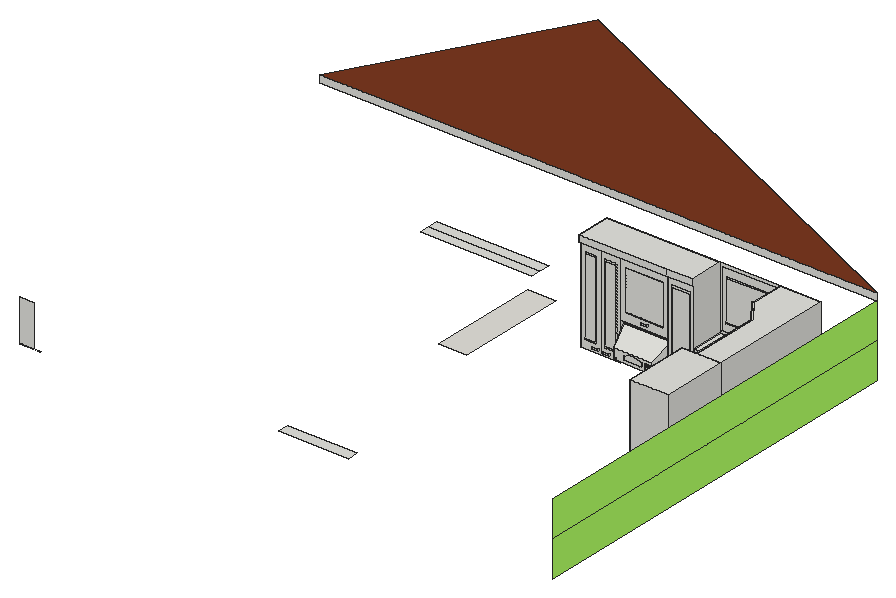
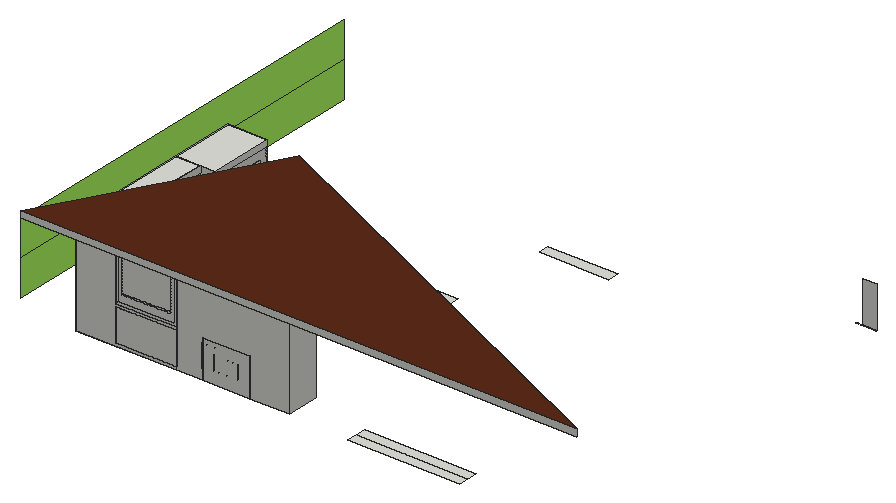
# SketchUp Ruby script. Lengths in inches.
U = 1.inch
M = Sketchup.active_model
def pt(a) = Geom::Point3d.new(a.map { |v| v * U })
def face(e, loops, mat)
  f = e.add_face(loops[0].map { |a| pt(a) })
  loops[1..].each { |l| e.add_face(l.map { |a| pt(a) }).erase! }
  f.material = f.back_material = mat if mat
  f
end
# faces: each face lists its corners as indices into pts; further lists are holes
def faces(e, pts, list, mat = nil) = list.each { |f| face(e, (f[0].is_a?(Array) ? f : [f]).map { |l| l.map { |i| pts[i] } }, mat) }
# xy, xz, yz: faces in a plane at the given z, y or x. An outline is a flat list of corners, or four numbers for a rectangle; further outlines are holes
def ring(l) = l.size == 4 ? [[l[0], l[1]], [l[2], l[1]], [l[2], l[3]], [l[0], l[3]]] : l.each_slice(2).to_a
def flat(e, list, mat, &to3) = list.each { |f| face(e, (f[0].is_a?(Array) ? f : [f]).map { |l| ring(l).map { |u, v| to3.(u, v) } }, mat) }
def xy(e, z, list, mat = nil) = flat(e, list, mat) { |x, y| [x, y, z] }
def xz(e, y, list, mat = nil) = flat(e, list, mat) { |x, z| [x, y, z] }
def yz(e, x, list, mat = nil) = flat(e, list, mat) { |y, z| [x, y, z] }
def lines(e, pts, list) = list.each { |a, b| e.add_line(pt(pts[a]), pt(pts[b])) }
# prism: a flat outline (further loops are holes) pulled along v
def prism(e, loops, v, mat = nil)
  f = face(e, loops, mat); d = Geom::Vector3d.new(v.map { |x| x * U })
  f.pushpull(f.normal.samedirection?(d) ? d.length : -d.length)
end
def box(e, o, s, mat = nil) = prism(e, [[o, [o[0] + s[0], o[1], o[2]], [o[0] + s[0], o[1] + s[1], o[2]], [o[0], o[1] + s[1], o[2]]]], [0, 0, s[2]], mat)
def at(x, y, z, deg = 0) = Geom::Transformation.translation(pt([x, y, z])) * Geom::Transformation.rotation(ORIGIN, Z_AXIS, deg.degrees)
def axes(o, x, y, z) = Geom::Transformation.new([*x, 0, *y, 0, *z, 0, *pt(o).to_a, 1])
def part(name) = M.definitions.add(name)
# library, detail: a bought-in or finely detailed component or shape, given as its bounding box
def library(name, o, s) = part(name).tap { |d| box(d.entities, o, s) }
def detail(e, o, s) = box(e.add_group.entities, o, s)
def put(e, d, t, mat = nil) = e.add_instance(d, t).tap { |i| i.material = mat if mat }
def group(e, t, mat = nil) = e.add_group.tap { |g| g.transformation = t; g.material = mat if mat }.entities
root = M.entities
M.materials.add("[Color F03]").color = [178, 255, 101]
M.materials.add("[Marble Carrara Gold Floor Tile]").color = [225, 223, 217]
M.materials.add("[Roofing Tile Spanish]").color = [138, 64, 36]
c1 = part("Countertop_Microwave\#1")
xy(c1.entities,0,[[0,0,20,15]])
xy(c1.entities,1.52,[[1.5,0,14.49,0.25]])
xy(c1.entities,9.5,[[1.5,0,14.49,0.25]])
xy(c1.entities,11,[[0,0,16.03,1.79],[16.03,0,20,1.79],[0,1.79,20,15]])
xz(c1.entities,0,[[[0,0,16.03,11],[0.875,0.875,15.15,10.125]],[[16.03,0,20,11],[16.98,2.6,19.1,7.06],[16.98,2.6,19.1,4.83],[16.98,8.23,16.98,9.51,17.18,9.61,17.38,9.6875,17.59,9.75,17.8,9.79,18.02,9.8125,18.24,9.8125,18.46,9.79,18.67,9.75,18.88,9.6875,19.08,9.61,19.28,9.51,19.28,8.23],[16.77,0.42,19.01,1.78],[16.98,5.95,19.1,7.06],[16.98,2.6,19.1,3.72],[16.98,4.83,19.1,5.39],[16.98,4.28,19.1,4.83]],[16.77,0.42,19.01,1.78],[[0.875,0.875,15.15,10.125],[1.5,1.52,14.49,9.5]],[16.98,2.6,19.1,3.72],
  [16.98,3.72,19.1,4.28],[16.98,4.28,19.1,4.83],[16.98,4.83,19.1,5.39],[16.98,5.39,19.1,5.95],[16.98,5.95,19.1,7.06],
  [16.98,8.23,19.28,8.23,19.28,9.51,19.08,9.61,18.88,9.6875,18.67,9.75,18.46,9.79,18.24,9.8125,18.02,9.8125,17.8,9.79,17.59,9.75,17.38,9.6875,17.18,9.61,16.98,9.51]])
xz(c1.entities,0.25,[[1.5,1.52,14.49,9.5]])
xz(c1.entities,15,[[0,0,20,11]])
yz(c1.entities,0,[[0,0,1.79,11],[1.79,0,15,11]])
yz(c1.entities,1.5,[[0,1.52,0.25,9.5]])
yz(c1.entities,14.49,[[0,1.52,0.25,9.5]])
yz(c1.entities,20,[[0,0,1.79,11],[1.79,0,15,11]])
p = [[18.04,0,5.95],[18.04,0,3.72],[18.57,0,5.95],[18.57,0,3.72],[17.51,0,5.95],[17.51,0,3.72]]
lines(c1.entities,p,[[0,1],[2,3],[4,5]])
c2 = part("Switch\#2")
xy(c2.entities,0,[[0,0,0.5,0.4]])
xz(c2.entities,0.81,[[0,0,0.5,0.15]])
yz(c2.entities,0,[[0.4,0,0.81,0.15,0.81,0]])
yz(c2.entities,0.5,[[0.4,0,0.81,0,0.81,0.15]])
p = [[0,0.81,0.15],[0,0.4,0],[0.5,0.4,0],[0.5,0.81,0.15]]
faces(c2.entities,p,[[0,1,2,3]])
c3 = part("Light")
xy(c3.entities,-1.25,[[1.75,0.12,2.49,0.16,3.16,0.49,3.65,1.05,3.88,1.75,3.84,2.49,3.51,3.16,2.95,3.65,2.25,3.88,1.51,3.84,0.84,3.51,0.35,2.95,0.12,2.25,0.16,1.51,0.49,0.84,1.05,0.35]])
xy(c3.entities,0,[[[1.74,0.02,2.52,0.07,3.22,0.41,3.73,1,3.98,1.74,3.93,2.52,3.59,3.22,3,3.73,2.26,3.98,1.48,3.93,0.78,3.59,0.27,3,0.02,2.26,0.07,1.48,0.41,0.78,1,0.27],[1.75,0.12,1.05,0.35,0.49,0.84,0.16,1.51,0.12,2.25,0.35,2.95,0.84,3.51,1.51,3.84,2.25,3.88,2.95,3.65,3.51,3.16,3.84,2.49,3.88,1.75,3.65,1.05,3.16,0.49,2.49,0.16]],[1.75,0.12,1.05,0.35,0.49,0.84,0.16,1.51,0.12,2.25,0.35,2.95,0.84,3.51,1.51,3.84,2.25,3.88,2.95,3.65,3.51,3.16,3.84,2.49,3.88,1.75,3.65,1.05,3.16,0.49,2.49,0.16]])
p = [[1.05,0.35,0],[1.75,0.12,0],[1.75,0.12,-1.25],[1.05,0.35,-1.25],[2.49,0.16,0],[2.49,0.16,-1.25],
  [3.16,0.49,0],[3.16,0.49,-1.25],[0.49,0.84,0],[0.49,0.84,-1.25],[3.65,1.05,0],[3.65,1.05,-1.25],
  [0.16,1.51,0],[0.16,1.51,-1.25],[3.88,1.75,0],[3.88,1.75,-1.25],[0.12,2.25,0],[0.12,2.25,-1.25],
  [3.84,2.49,0],[3.84,2.49,-1.25],[0.35,2.95,0],[0.35,2.95,-1.25],[3.51,3.16,0],[3.51,3.16,-1.25],
  [0.84,3.51,0],[0.84,3.51,-1.25],[2.95,3.65,0],[2.95,3.65,-1.25],[1.51,3.84,0],[1.51,3.84,-1.25],
  [2.25,3.88,0],[2.25,3.88,-1.25]]
faces(c3.entities,p,[[0,1,2,3],[1,4,5,2],[4,6,7,5],[8,0,3,9],[6,10,11,7],[12,8,9,13],[10,14,15,11],[16,12,13,17],
  [14,18,19,15],[20,16,17,21],[18,22,23,19],[24,20,21,25],[22,26,27,23],[28,24,25,29],[26,30,31,27],[30,28,29,31]])
c4 = part("Hood_UnderCabinet_32in \#1")
xy(c4.entities,0,[[[0,-7,32,0],[8,-6.5,24,-2.1875]]])
xy(c4.entities,12,[[[0,-7,32,0],[8,-6.5,24,-2.1875]],[8,-6.5,24,-2.1875]])
xy(c4.entities,20,[[[3,-7,29,-3.6875],[10,-6.03,10,-5.03,11.97,-4.57,13.98,-4.3,16,-4.2,18.02,-4.3,20.03,-4.57,22,-5.03,22,-6.03],[24.44,-6.01,28.38,-4.7],[3.24,-6.76,4.74,-6.19]]])
xy(c4.entities,20.1875,[[3.24,-6.76,4.74,-6.19],[10,-6.03,22,-6.03,22,-5.03,20.03,-4.57,18.02,-4.3,16,-4.2,13.98,-4.3,11.97,-4.57,10,-5.03],[[24.44,-6.01,28.38,-4.7],[27.58,-5.75,27.48,-5.74,27.39,-5.7,27.32,-5.64,27.26,-5.57,27.22,-5.48,27.21,-5.38,27.22,-5.28,27.26,-5.19,27.32,-5.11,27.39,-5.05,27.48,-5.02,27.58,-5,27.68,-5.02,27.77,-5.05,27.85,-5.11,27.91,-5.19,27.94,-5.28,27.96,-5.38,27.94,-5.48,27.91,-5.57,27.85,-5.64,27.77,-5.7,27.68,-5.74]],[27.58,-5.75,27.48,-5.74,27.39,-5.7,27.32,-5.64,27.26,-5.57,27.22,-5.48,27.21,-5.38,27.22,-5.28,27.26,-5.19,27.32,-5.11,27.39,-5.05,27.48,-5.02,27.58,-5,27.68,-5.02,27.77,-5.05,27.85,-5.11,27.91,-5.19,27.94,-5.28,27.96,-5.38,27.94,-5.48,27.91,-5.57,27.85,-5.64,27.77,-5.7,27.68,-5.74],[27.58,-5.75,27.48,-5.74,27.39,-5.7,27.32,-5.64,27.26,-5.57,27.22,-5.48,27.21,-5.38,27.22,-5.28,27.26,-5.19,27.32,-5.11,27.39,-5.05,27.48,-5.02,27.58,-5,27.68,-5.02,27.77,-5.05,27.85,-5.11,27.91,-5.19,27.94,-5.28,27.96,-5.38,27.94,-5.48,27.91,-5.57,27.85,-5.64,27.77,-5.7,27.68,-5.74]])
xz(c4.entities,-7,[[0,12,32,12,29,20,3,20]])
xz(c4.entities,-6.76,[[3.24,20,4.74,20.1875]])
xz(c4.entities,-6.5,[[[8,0,24,12],[9.12,1.55,22.92,11.3]],[[9.12,1.55,22.92,11.3],[9.62,2.05,22.42,10.8]],[9.62,2.05,22.42,10.8]])
xz(c4.entities,-6.19,[[3.24,20,4.74,20.1875]])
xz(c4.entities,-6.03,[[10,20,22,20.1875]])
xz(c4.entities,-6.01,[[24.44,20,28.38,20.1875]])
xz(c4.entities,-4.7,[[24.44,20,28.38,20.1875]])
xz(c4.entities,-2.1875,[[8,0,24,12]])
xz(c4.entities,0,[[0,0,32,12]])
yz(c4.entities,0,[[-7,0,0,12]])
yz(c4.entities,3.24,[[-6.76,20,-6.19,20.1875]])
yz(c4.entities,4.74,[[-6.76,20,-6.19,20.1875]])
yz(c4.entities,8,[[-6.5,0,-2.1875,12]])
yz(c4.entities,10,[[-6.03,20,-5.03,20.1875]])
yz(c4.entities,22,[[-6.03,20,-5.03,20.1875]])
yz(c4.entities,24,[[-6.5,0,-2.1875,12]])
yz(c4.entities,24.44,[[-6.01,20,-4.7,20.1875]])
yz(c4.entities,28.38,[[-6.01,20,-4.7,20.1875]])
yz(c4.entities,32,[[-7,0,0,12]])
p = [[0,-7,12],[3,-7,20],[3,-3.6875,20],[0,0,12],[29,-7,20],[32,-7,12],
  [32,0,12],[29,-3.6875,20],[11.97,-4.57,20],[10,-5.03,20],[10,-5.03,20.1875],[11.97,-4.57,20.1875],
  [22,-5.03,20],[20.03,-4.57,20],[20.03,-4.57,20.1875],[22,-5.03,20.1875],[13.98,-4.3,20],[13.98,-4.3,20.1875],
  [18.02,-4.3,20],[18.02,-4.3,20.1875],[16,-4.2,20],[16,-4.2,20.1875]]
faces(c4.entities,p,[[0,1,2,3],[4,5,6,7],[2,7,6,3],[8,9,10,11],[12,13,14,15],[16,8,11,17],[13,18,19,14],[20,16,17,21],
  [18,20,21,19]])
put(c4.entities,c2,at(25.49,-5.75,20.1875))
put(c4.entities,c2,at(24.74,-5.75,20.1875))
put(c4.entities,c3,axes([22,-7,14],[1,0,0],[0,0,1],[0,-1,0]))
put(c4.entities,c2,at(26.24,-5.75,20.1875))
put(c4.entities,c3,axes([6,-7,14],[1,0,0],[0,0,1],[0,-1,0]))
c5 = part("quarter")
xy(c5.entities,0,[[1.5,0,1.5,0.25,1.75,0.67,2.17,0.91,2.41,0.91,2.41,0]])
p = [[1.5,0.25,0],[1.5,0,0],[0.83,0,0.29],[0.83,0.43,0.29],[1.25,1.16,0.29],[1.75,0.67,0],
  [1.99,1.59,0.29],[2.17,0.91,0],[2.41,1.59,0.29],[2.41,0.91,0],[0.3,0,0.8125],[0.3,0.57,0.8125],
  [0.87,1.55,0.8125],[1.85,2.11,0.8125],[2.41,2.11,0.8125],[0,0,1.5],[0,0.65,1.5],[0.65,1.77,1.5],
  [1.77,2.41,1.5],[2.41,2.41,1.5]]
faces(c5.entities,p,[[0,1,2,3],[4,5,0,3],[6,7,5,4],[6,8,9,7],[3,2,10,11],[12,4,3,11],[13,6,4,12],[13,14,8,6],
  [11,10,15,16],[17,12,11,16],[18,13,12,17],[18,19,14,13]])
c6 = part("Dishes_Bowl_5in")
put(c6.entities,c5,at(-2.41,0,0.125))
put(c6.entities,c5,at(0,2.41,0.125,-90))
put(c6.entities,c5,at(0,-2.41,0.125,90))
put(c6.entities,c5,at(2.41,0,0.125,-180))
xy(root,114.79,[[208.97,349.92,225.68,378.03],[215.59,378.03,215.59,417.74,182.47,417.74,182.47,431.8,225.68,431.8,225.68,378.03],[215.59,407.7,208.39,417.74,215.59,417.74]])
xy(root,115.79,[[143.2,417.42,146.05,417.74]])
xy(root,115.89,[[208.97,350.72,225.68,377.22]])
xy(root,116.02,[[138.46,417.42,141.31,417.74]])
xy(root,116.04,[[215.36,388.03,215.59,392.01]])
xy(root,116.09,[[215.36,393.61,215.59,397.59]])
xy(root,116.18,[[171.98,417.42,174.83,417.74]])
xy(root,116.34,[[143.2,417.42,146.05,417.74]])
xy(root,116.56,[[138.46,417.42,141.31,417.74]])
xy(root,116.59,[[215.36,388.03,215.59,392.01]])
xy(root,116.64,[[215.36,393.61,215.59,397.59]])
xy(root,116.73,[[171.98,417.42,174.83,417.74]])
xy(root,122.43,[[99,298.5,129,303],[50.67,435,98.67,439.5],[50.67,439.5,98.67,444]])
xy(root,130.07,[[182.47,417.74,208.39,431.8]])
xy(root,131.16,[[150.78,417.74,170.95,431.8],[182.47,417.74,208.39,431.8]])
xy(root,132.6875,[[159.55,417.42,162.4,417.74]])
xy(root,133.23,[[159.55,417.42,162.4,417.74]])
xy(root,134.43,[[117,361.98,129,409.98]],"[Marble Carrara Gold Floor Tile]")
xy(root,135.52,[[208.97,350.72,225.68,377.22]])
xy(root,155.7,[[215.02,378.03,215.02,407.37,207.99,417.18,208.39,417.74,215.59,407.7,215.59,378.03],[133.5,416.94,145.02,417.74],[145.02,416.94,170.95,417.74],[170.95,416.94,182.47,417.74],[145.02,417.74,170.95,431.4]])
xy(root,155.92,[[145.02,417.74,170.95,431.4]])
xy(root,158.43,[[208.97,349.92,225.68,378.03],[215.02,378.03,215.59,378.03,215.59,407.7,208.39,417.74,207.99,417.18,215.02,407.37],[215.59,378.03,225.68,378.03,225.68,431.8,208.39,431.8,208.39,417.74,215.59,407.7],[133.5,416.94,182.47,431.8]])
xz(root,282.68,[[0,128.43,9,128.43,6,128.44,0,128.44],[0,128.44,6,146.43]])
xz(root,349.92,[[208.97,114.79,225.68,158.43]])
xz(root,350.72,[[208.97,115.89,225.68,135.52]])
xz(root,377.22,[[208.97,115.89,225.68,135.52]])
xz(root,378.03,[[208.97,114.79,208.97,158.43,215.02,158.43,215.02,155.7,215.59,155.7,215.59,114.79],[215.59,114.79,225.68,158.43],[215.02,155.7,215.59,158.43]])
xz(root,388.03,[[215.36,116.04,215.59,116.59]])
xz(root,392.01,[[215.36,116.04,215.59,116.59]])
xz(root,393.61,[[215.36,116.09,215.59,116.64]])
xz(root,397.59,[[215.36,116.09,215.59,116.64]])
xz(root,416.94,[[133.5,155.7,170.95,158.43],[170.95,155.7,182.47,158.43]])
xz(root,417.42,[[143.2,115.79,146.05,116.34],[138.46,116.02,141.31,116.56],[171.98,116.18,174.83,116.73],[159.55,132.6875,162.4,133.23]])
xz(root,417.74,[[[133.5,114.79,142.14,155.7],[135.23,118.07,140.41,152.43],[138.46,116.02,141.31,116.56]],[[142.14,114.79,150.78,155.7],[143.87,118.07,149.05,152.43],[143.2,115.79,146.05,116.34]],[[170.95,114.79,182.47,155.7],[172.68,118.07,180.74,152.43],[171.98,116.18,174.83,116.73]],[182.47,114.79,208.39,116.05],[[135.23,118.07,140.41,152.43],[135.52,118.61,140.125,151.89]],
  [[143.87,118.07,149.05,152.43],[144.16,118.61,148.77,151.89]],[[172.68,118.07,180.74,152.43],[172.96,118.61,180.45,151.89]],[135.52,118.61,140.125,151.89],[144.16,118.61,148.77,151.89],[172.96,118.61,180.45,151.89],
  [182.47,130.07,208.39,131.16],[[150.78,131.16,170.95,155.7],[152.51,134.43,169.22,152.43],[159.55,132.6875,162.4,133.23]],[[152.51,134.43,169.22,152.43],[152.8,134.98,168.93,151.89]],[152.8,134.98,168.93,151.89],[145.02,155.7,170.95,155.92]])
xz(root,431.4,[[145.02,155.7,170.95,155.92]])
xz(root,431.8,[[133.5,114.79,133.5,158.43,182.47,158.43,182.47,114.79,170.95,114.79,170.95,131.16,150.78,131.16,150.78,114.79],[150.78,114.79,170.95,131.16],[182.47,114.79,182.47,115.89,208.39,115.89,208.39,130.07,182.47,130.07,182.47,131.16,208.39,131.16,208.39,158.43,225.68,158.43,225.68,114.79],[182.47,115.89,208.39,130.07],[[182.47,131.16,208.39,158.43],[183.04,132.25,207.82,157.34]],
  [[183.04,132.25,207.82,157.34],[184.77,135.52,206.09,154.07]],[[184.77,135.52,206.09,154.07],[185.0625,136.07,205.8,153.52]],[185.0625,136.07,205.8,153.52]])
xz(root,444,[[0,158.43,240,161.43]])
xz(root,444,[[0,161.43,120,224.68,240,161.43]],"[Roofing Tile Spanish]")
yz(root,133.5,[[417.74,114.79,431.8,114.79,431.8,158.43,416.94,158.43,416.94,155.7,417.74,155.7]])
yz(root,138.46,[[417.42,116.02,417.74,116.56]])
yz(root,141.31,[[417.42,116.02,417.74,116.56]])
yz(root,143.2,[[417.42,115.79,417.74,116.34]])
yz(root,145.02,[[417.74,155.7,431.4,155.92]])
yz(root,146.05,[[417.42,115.79,417.74,116.34]])
yz(root,150.78,[[417.74,114.79,431.8,131.16]])
yz(root,159.55,[[417.42,132.6875,417.74,133.23]])
yz(root,162.4,[[417.42,132.6875,417.74,133.23]])
yz(root,170.95,[[417.74,114.79,431.4,131.16],[431.4,114.79,431.8,131.16],[417.74,131.16,431.4,155.7],[417.74,155.7,431.4,155.92]])
yz(root,171.98,[[417.42,116.18,417.74,116.73]])
yz(root,174.83,[[417.42,116.18,417.74,116.73]])
yz(root,182.47,[[431.8,115.89,431.8,130.07,417.74,130.07,417.74,116.05],[417.74,130.07,431.8,131.16],[417.74,131.16,431.8,131.16,431.8,158.43,416.94,158.43,416.94,155.7,417.74,155.7]])
yz(root,208.39,[[431.8,115.89,417.74,116.05,417.74,130.07,431.8,130.07],[417.74,131.16,431.8,158.43]])
yz(root,208.97,[[[349.92,114.79,378.03,136.61],[350.72,115.89,377.22,135.52]],[349.92,136.61,350.72,155.7],[[350.72,136.61,377.22,155.7],[353.13,139.89,374.81,152.43]],[377.22,136.61,378.03,155.7],[[353.13,139.89,374.81,152.43],[353.53,140.43,374.41,151.89]],
  [353.53,140.43,374.41,151.89],[349.92,155.7,378.03,158.43]])
yz(root,215.02,[[378.03,155.7,407.37,158.43]])
yz(root,215.36,[[388.03,116.04,392.01,116.59],[393.61,116.09,397.59,116.64]])
yz(root,215.59,[[[378.03,114.79,392.87,155.7],[380.4375,118.07,390.46,152.43],[388.03,116.04,392.01,116.59]],[[392.87,114.79,407.7,155.7],[395.27,118.07,405.29,152.43],[393.61,116.09,397.59,116.64]],[[380.4375,118.07,390.46,152.43],[380.84,118.61,390.05,151.89]],[[395.27,118.07,405.29,152.43],[395.68,118.61,404.89,151.89]],[380.84,118.61,390.05,151.89],
  [395.68,118.61,404.89,151.89]])
yz(root,225.68,[[[349.92,114.79,378.03,158.43],[350.72,115.89,377.22,135.52]],[378.03,114.79,431.8,158.43]])
yz(root,240,[[269.63,127.68,444,143.06],[269.63,143.06,444,158.43]],"[Color F03]")
p = [[215.59,407.7,114.79],[215.59,407.7,155.7],[208.39,417.74,155.7],[208.39,417.74,131.16],[208.39,417.74,130.07],[208.39,417.74,116.05],
  [208.39,417.74,114.79],[209.62,416.04,118.07],[209.62,416.04,130.07],[209.62,416.04,131.16],[209.62,416.04,152.43],[214.37,409.41,152.43],
  [214.37,409.41,118.07],[208.39,431.8,115.89],[182.47,431.8,115.89],[182.47,417.74,116.05],[214.17,409.69,118.61],[209.82,415.76,118.61],
  [209.82,415.76,130.07],[209.82,415.76,131.16],[209.82,415.76,151.89],[214.17,409.69,151.89],[215.02,407.37,155.7],[215.02,407.37,158.43],
  [207.99,417.18,158.43],[207.99,417.18,155.7],[208.39,417.74,158.43]]
faces(root,p,[[[0,1,2,3,4,5,6],[7,8,9,10,11,12]],[5,13,14,15],[[8,7,12,11,10,9],[16,17,18,19,20,21]],[17,16,21,20,19,18],[22,23,24,25],[24,26,2,25]])
put(root,c1,axes([210.28,374.56,115.89],[0,-1.02,0],[0.73165,0,0],[0,0,1.38545]))
put(root,c4,axes([150.78,431.8,129.18],[0.64385,0,0],[0,0,1.38545],[0,-1.02,0]))
put(root,c6,axes([195.98,422.73,115.99],[-0.73165,0,0],[0,-1.01996,0.01192],[0,0.01619,1.38534]))
put(root,c6,axes([188.21,422.74,115.99],[-0.73165,0,0],[0,-1.01996,0.01192],[0,0.01619,1.38534]))
put(root,c6,axes([203.42,422.92,115.99],[-1.13406,0,0],[0,-1.58094,0.01848],[0,0.0251,2.14727]))
